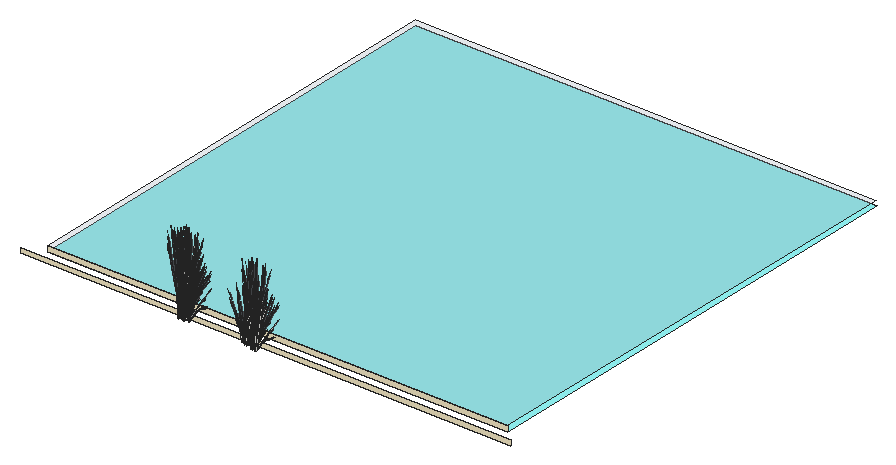
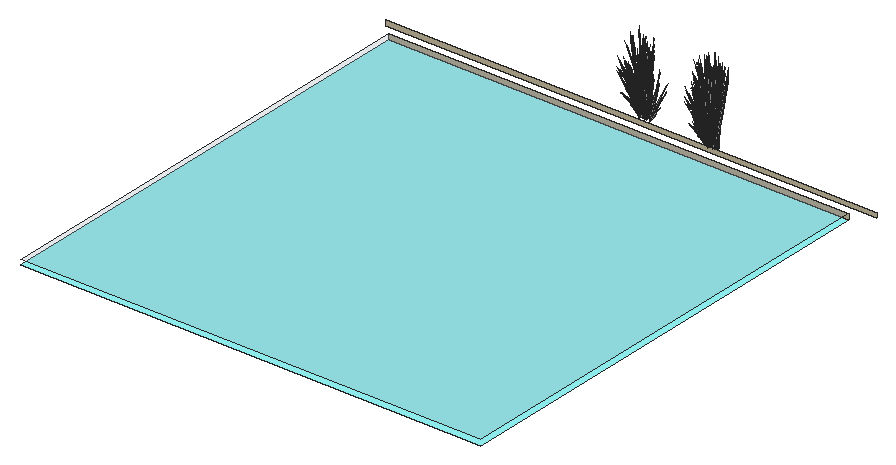
# SketchUp Ruby script. Lengths in inches.
U = 1.inch
M = Sketchup.active_model
def pt(a) = Geom::Point3d.new(a.map { |v| v * U })
def face(e, loops, mat)
  f = e.add_face(loops[0].map { |a| pt(a) })
  loops[1..].each { |l| e.add_face(l.map { |a| pt(a) }).erase! }
  f.material = f.back_material = mat if mat
  f
end
# faces: each face lists its corners as indices into pts; further lists are holes
def faces(e, pts, list, mat = nil) = list.each { |f| face(e, (f[0].is_a?(Array) ? f : [f]).map { |l| l.map { |i| pts[i] } }, mat) }
# xy, xz, yz: faces in a plane at the given z, y or x. An outline is a flat list of corners, or four numbers for a rectangle; further outlines are holes
def ring(l) = l.size == 4 ? [[l[0], l[1]], [l[2], l[1]], [l[2], l[3]], [l[0], l[3]]] : l.each_slice(2).to_a
def flat(e, list, mat, &to3) = list.each { |f| face(e, (f[0].is_a?(Array) ? f : [f]).map { |l| ring(l).map { |u, v| to3.(u, v) } }, mat) }
def xy(e, z, list, mat = nil) = flat(e, list, mat) { |x, y| [x, y, z] }
def xz(e, y, list, mat = nil) = flat(e, list, mat) { |x, z| [x, y, z] }
def yz(e, x, list, mat = nil) = flat(e, list, mat) { |y, z| [x, y, z] }
def lines(e, pts, list) = list.each { |a, b| e.add_line(pt(pts[a]), pt(pts[b])) }
# prism: a flat outline (further loops are holes) pulled along v
def prism(e, loops, v, mat = nil)
  f = face(e, loops, mat); d = Geom::Vector3d.new(v.map { |x| x * U })
  f.pushpull(f.normal.samedirection?(d) ? d.length : -d.length)
end
def box(e, o, s, mat = nil) = prism(e, [[o, [o[0] + s[0], o[1], o[2]], [o[0] + s[0], o[1] + s[1], o[2]], [o[0], o[1] + s[1], o[2]]]], [0, 0, s[2]], mat)
def at(x, y, z, deg = 0) = Geom::Transformation.translation(pt([x, y, z])) * Geom::Transformation.rotation(ORIGIN, Z_AXIS, deg.degrees)
def axes(o, x, y, z) = Geom::Transformation.new([*x, 0, *y, 0, *z, 0, *pt(o).to_a, 1])
def part(name) = M.definitions.add(name)
# library, detail: a bought-in or finely detailed component or shape, given as its bounding box
def library(name, o, s) = part(name).tap { |d| box(d.entities, o, s) }
def detail(e, o, s) = box(e.add_group.entities, o, s)
def put(e, d, t, mat = nil) = e.add_instance(d, t).tap { |i| i.material = mat if mat }
def group(e, t, mat = nil) = e.add_group.tap { |g| g.transformation = t; g.material = mat if mat }.entities
root = M.entities
M.materials.add("D01_Frost_White").color = [255, 242, 206]
M.materials.add("Glass_Basic_01").color = [161, 173, 186]
M.materials["Glass_Basic_01"].alpha = 0.25
M.materials.add("H02_Aqua_Frost").color = [153, 255, 255]
M.materials.add("LightPink_Translucent").color = [144, 107, 117]
M.materials["LightPink_Translucent"].alpha = 0.75
c1 = part("blade")
p = [[2.15,0.21,22],[0,0.17,0],[0.09,0.45,0],[2.18,0.31,22],[2.29,0.31,22],[0.38,0.45,0],
  [2.48,0.24,33],[2.49,0.24,33],[2.48,0.22,33]]
faces(c1.entities,p,[[0,1,2,3],[4,5,2,3],[6,3,4,7],[8,0,3,6]])
c2 = part("seeds")
p = [[0.3,-0.1,1.38],[-0.01,-0.03,1.59],[-0.01,-0.03,0.03],[0.14,-0.07,-0.07],[0.29,-0.03,3],[0.15,0.01,3.11]]
faces(c2.entities,p,[[0,1,2,3],[1,0,4,5]],"LightPink_Translucent")
c3 = part("blade with seeds")
put(c3.entities,c1,at(0,0,0))
put(c3.entities,c2,axes([2.4,0.25,30.99],[1.5799,-0.05474,1.17369],[-0.12525,1.92788,0.29478],[-0.07173,-0.02425,1.56792]))
xy(root,0,[[666.12,288,846,468]],"H02_Aqua_Frost")
xy(root,2,[[666.12,288,846,468]],"Glass_Basic_01")
xz(root,282,[[660.12,0,852,2]],"D01_Frost_White")
xz(root,288,[[666.12,0,846,2]],"D01_Frost_White")
put(root,c3,axes([724.84,280.2,1.22],[0.1218,-0.38743,-0.11714],[0.57753,0.06753,0.25635],[-0.10091,-0.0535,0.7822]))
put(root,c3,axes([753.51,278.125,1.11],[-0.49904,0.02018,-0.2237],[-0.04513,-0.33504,0.10766],[-0.08934,0.03396,0.71822]))
put(root,c3,axes([755.85,278.29,1.3],[-0.11068,-0.08041,0.71501],[0.144,-0.26601,-0.15377],[0.22393,0.03604,0.3057]))
put(root,c3,axes([753.875,278.58,1.1],[0.4633,0.14679,0],[-0.22297,0.30501,0],[0,0,0.87477]))
put(root,c3,axes([724.87,279.54,1.36],[-0.49904,0.02018,0.2237],[-0.04513,-0.33504,-0.10766],[0.08934,-0.03396,0.71822]))
put(root,c3,axes([723.58,279.78,1.24],[0,0.32696,0.24825],[-0.51416,0,0],[0,-0.07447,0.78752]))
put(root,c3,axes([727.21,280.11,2.52],[-0.23123,-0.29606,-0.0608],[0.41039,-0.14549,-0.33747],[0.17294,-0.03906,0.51278]))
put(root,c3,axes([727.19,279.86,2.34],[0.1245,-0.29741,-0.25549],[0.42685,0.10194,-0.1979],[0.17186,-0.02727,0.48886]))
put(root,c3,axes([755.22,278.41,2.36],[0.09858,-0.00553,0.87472],[0.2704,-0.25401,-0.13834],[0.17535,0.03353,0.07015]))
put(root,c3,axes([754.06,278.9,1.1],[-0.28374,-0.32877,-0.02571],[0.4807,-0.18271,0.25804],[-0.11845,0.0313,0.81815]))
put(root,c3,axes([726.52,278.64,1.1875],[0.28732,-0.32763,0],[0.4807,0.18271,-0.25804],[0.10948,0.04161,0.81856]))
put(root,c3,axes([753.96,278.11,1.31],[0.33952,0.19644,0.0724],[-0.2832,0.22163,-0.20674],[-0.07883,0.02996,0.63372]))
put(root,c3,axes([724.8,280.05,1.11],[-0.27607,-0.27443,-0.2237],[0.41817,-0.19325,0.10766],[-0.08934,-0.03396,0.71822]))
put(root,c3,axes([724.85,279.66,1.18],[0.1998,0.3656,0.22877],[-0.5709,0.12713,0.08977],[0.00698,-0.06718,0.79428]))
put(root,c3,axes([751.28,278.16,2.37],[-0.11397,-0.30091,0.24001],[0.44709,-0.05222,0.1979],[-0.13177,0.07077,0.49665]))
put(root,c3,axes([751.1875,278.1,2.37],[-0.31549,-0.13751,0.03215],[0.18368,-0.19581,0.2531],[-0.10115,0.06331,0.38595]))
put(root,c3,axes([751.33,277.74,1.9375],[0.15946,-0.06916,0.85688],[0.13424,0.31957,0.06928],[-0.25033,0.07223,0.36631]))
put(root,c3,axes([727.65,279.9375,0.99],[-0.29599,0.03924,0.70792],[-0.04711,-0.31232,0.04052],[0.20731,-0.04727,0.40283]))
put(root,c3,axes([728.1875,279.66,1.13],[-0.28491,-0.20907,-0.03244],[0.31204,-0.19157,-0.14708],[0.08842,-0.01349,0.48512]))
put(root,c3,axes([724.75,279.95,1.36],[-0.22297,0.29461,0.2237],[-0.4633,-0.14179,-0.10766],[0,-0.06791,0.71822]))
put(root,c3,axes([725.57,279.69,1.1],[0,-0.37831,0],[0.57465,0,0],[0,0,0.89728]))
put(root,c3,axes([754.84,278.45,2.49],[0.45939,0.00787,-0.35523],[-0.03085,0.3315,0.04287],[0.19462,0.03498,0.5025]))
put(root,c3,axes([726.27,278.82,1.24],[-0.4301,-0.16348,0.24825],[0.25708,-0.29314,0],[0.09796,0.03723,0.78752]))
put(root,c3,axes([727.11,279.96,2.49],[0.40382,-0.1444,-0.35523],[0.22505,0.29724,0.04287],[0.19512,-0.03377,0.5025]))
put(root,c3,axes([754.32,278.71,1.24],[0.4301,-0.16348,0.24825],[0.25708,0.29314,0],[-0.09796,0.03723,0.78752]))
put(root,c3,axes([753.71,278.46,1.15],[0.1998,0.37562,-0.03006],[-0.5709,0.13162,0],[0.00698,0.01312,0.86086]))
put(root,c3,axes([753.93,278.86,1.01],[-0.42874,-0.0809,-0.15489],[0.10795,-0.28489,0.15489],[-0.08643,0.03285,0.69487]))
put(root,c3,axes([725.3,279.45,1.18],[-0.38104,0.29672,0.22877],[-0.45269,-0.26192,0.08977],[0.09186,-0.02961,0.79428]))
put(root,c3,axes([750.84,278.28,1.3],[0.15971,0.02684,0.71501],[0.10294,0.27415,-0.15377],[-0.21694,0.05132,0.3057]))
put(root,c3,axes([725.72,279.98,1.15],[-0.42746,-0.28142,-0.03066],[0.42772,-0.28159,0],[-0.01493,-0.00983,0.87786]))
put(root,c3,axes([751.55,278.06,2.53],[0.40003,-0.04673,0.17707],[0.10563,0.26712,-0.2286],[-0.11464,0.07175,0.4374]))
put(root,c3,axes([755.59,277.78,1.1875],[0.57465,0,0],[0,0.36542,-0.25804],[0,0.08323,0.81856]))
put(root,c3,axes([724.64,278.96,1.24],[-0.13276,0.32494,0.08821],[-0.4858,-0.09195,0.17543],[0.08392,-0.00158,0.80203]))
put(root,c3,axes([750.01,277.94,2.35],[0.05865,0.00877,0.88692],[0.18143,0.28888,-0.08381],[-0.12006,0.07582,0.15695]))
put(root,c3,axes([755.36,277.96,1.1],[-0.57436,-0.00261,-0.02488],[0,-0.36542,0.24971],[-0.01805,0.08319,0.79176]))
put(root,c3,axes([727.05,280.02,2.53],[-0.38192,-0.09121,0.17707],[0.11139,-0.2661,-0.2286],[0.15377,-0.0244,0.4374]))
put(root,c3,axes([754.11,277.65,1.33],[0.51755,0.15601,-0.14548],[-0.2492,0.32927,-0.25001],[0.01626,0.08084,0.79854]))
put(root,c3,axes([724.4375,279.23,0.8],[-0.45234,0.1309,0.64464],[-0.14398,-0.37559,0.25048],[0.27777,0.00625,0.73321]))
put(root,c3,axes([750.5,278.86,1.38],[0.19152,-0.14818,0.5743],[0.07557,0.23459,0.42196],[-0.13841,0.042,0.12649]))
put(root,c3,axes([755.11,278.58,2.26],[0.26148,0.20471,-0.17707],[-0.29857,0.19378,0.2286],[0.1517,0.02948,0.4374]))
put(root,c3,axes([725.65,279.32,1.31],[0.08866,-0.29179,0.0724],[0.43315,0.05065,-0.20674],[0.07883,0.02996,0.63372]))
put(root,c3,axes([755.24,278.02,1.01],[-0.32079,0.20399,-0.15489],[-0.32079,-0.20399,0.15489],[0,0.06571,0.69487]))
put(root,c3,axes([753.86,278.04,1.33],[0.05355,0.37308,-0.14548],[-0.55775,0.02256,-0.25001],[-0.09822,0.04969,0.79854]))
put(root,c3,axes([754.98,278.66,2.37],[-0.02314,0.24862,0.03215],[-0.34943,-0.00682,0.2531],[0.13385,0.02602,0.38595]))
put(root,c3,axes([754.06,277.89,1.11],[-0.22297,0.29461,-0.2237],[-0.4633,-0.14179,0.10766],[0,0.06791,0.71822]))
put(root,c3,axes([724.9,280.02,1.18],[0.58084,0.06889,0.22877],[-0.11821,0.38906,0.08977],[-0.08488,-0.03757,0.79428]))
put(root,c3,axes([727.97,279.73,0.75],[-0.02402,-0.04964,0.88171],[0.16658,-0.29036,-0.1347],[0.16804,-0.00418,0.15018]))
put(root,c3,axes([751.23,278.22,2.26],[-0.40003,0.04673,-0.17707],[-0.10563,-0.26712,0.2286],[-0.11464,0.07175,0.4374]))
put(root,c3,axes([755.01,278.58,2.37],[-0.33886,0.21544,0.24001],[-0.29224,-0.22879,0.1979],[0.15898,0.03974,0.49665]))
put(root,c3,axes([725.47,279.4,1.36],[-0.27607,-0.27443,0.2237],[0.41817,-0.19325,-0.10766],[0.08934,0.03396,0.71822]))
put(root,c3,axes([724.04,280.66,1.01],[-0.10795,-0.28489,-0.15489],[0.42874,-0.0809,0.15489],[-0.08643,-0.03285,0.69487]))
put(root,c3,axes([724.59,280.64,1.24],[0.49383,-0.08678,0.08821],[0.12194,0.32295,0.17543],[-0.04404,-0.04705,0.80203]))
put(root,c3,axes([725.61,279.42,1.33],[0.46399,-0.21707,-0.14548],[0.30855,0.30672,-0.25001],[0.11448,0.03115,0.79854]))
put(root,c3,axes([727.45,279.99,2.26],[0.38192,0.09121,-0.17707],[-0.11139,0.2661,0.2286],[0.15377,-0.0244,0.4374]))
put(root,c3,axes([750.64,278.82,2.82],[0.40553,0.08728,-0.03244],[-0.12475,0.26862,-0.14708],[-0.06633,0.04078,0.48512]))
put(root,c3,axes([753.52,278.32,1.03],[-0.30954,0.24575,-0.31177],[-0.38452,-0.22284,-0.08182],[-0.12404,0.0613,0.68817]))
put(root,c3,axes([753.93,278.83,2.53],[-0.07098,-0.26335,0.17707],[0.40574,-0.06954,-0.2286],[0.10898,0.07547,0.4374]))
put(root,c3,axes([726.78,278.84,1.01],[0.4301,0.16348,-0.24825],[-0.25708,0.29314,0],[0.09796,0.03723,0.78752]))
put(root,c3,axes([754.07,278.73,1.17],[0.57533,0.10627,0.15378],[-0.14394,0.37986,-0.18246],[-0.09522,0.04754,0.82443]))
put(root,c3,axes([754.03,278.99,1.01],[-0.4301,0.16348,-0.24825],[-0.25708,-0.29314,0],[-0.09796,0.03723,0.78752]))
put(root,c3,axes([755.46,278.02,1.01],[0,0.32696,-0.24825],[-0.51416,0,0],[0,0.07447,0.78752]))
put(root,c3,axes([725.96,279.77,1.1],[0.51416,0,0],[0,0.33849,0],[0,0,0.89203]))
put(root,c3,axes([754.17,278.06,1.9375],[-0.1707,-0.05633,0.85688],[0.35326,-0.23632,0.06928],[0.22018,0.10661,0.36631]))
put(root,c3,axes([725.09,280.2,1.33],[-0.46399,0.21707,-0.14548],[-0.30855,-0.30672,-0.25001],[-0.11448,-0.03115,0.79854]))
put(root,c3,axes([726.11,278.98,1.24],[-0.49383,0.08678,0.08821],[-0.12194,-0.32295,0.17543],[0.04404,0.04705,0.80203]))
put(root,c3,axes([754.21,277.32,2.24],[-0.39711,-0.16988,0.69141],[0.41931,-0.2645,0.29833],[0.12812,0.1594,0.66832]))
put(root,c3,axes([726.41,279.66,1.9375],[-0.19062,0.00741,0.85688],[0.12645,-0.32094,0.06928],[0.27165,0.01985,0.36631]))
put(root,c3,axes([726.66,278.96,1.01],[0.10795,0.28489,-0.15489],[-0.42874,0.0809,0.15489],[0.08643,0.03285,0.69487]))
put(root,c3,axes([751.34,278.04,2.52],[0.4251,0.18028,-0.0608],[-0.24491,0.26108,-0.33747],[-0.1201,0.09075,0.51278]))
put(root,c3,axes([754.81,278.7,1.38],[-0.25875,-0.09401,0.5743],[0.33411,-0.09552,0.42196],[0.09012,0.08091,0.12649]))
put(root,c3,axes([753.9,278.97,2.52],[0.27385,-0.27986,-0.0608],[0.39658,0.16123,-0.33747],[0.13785,0.07907,0.51278]))
put(root,c3,axes([727.4,280.1,2.37],[0.16879,0.22293,0.03215],[-0.30779,0.10912,0.2531],[0.13568,-0.02153,0.38595]))
put(root,c3,axes([751.92,277.95,1.9375],[0.11478,-0.10046,0.85688],[0.28982,0.27117,0.06928],[-0.19878,0.12349,0.36631]))
put(root,c3,axes([725.8,279.6,1.19],[-0.58084,-0.06889,0.24599],[0.11821,-0.38906,0.09653],[0.08488,0.03757,0.85407]))
put(root,c3,axes([727.36,280.02,2.37],[-0.12984,0.29812,0.24001],[-0.42685,-0.10194,0.1979],[0.16786,-0.01792,0.49665]))
put(root,c3,axes([725.33,280.5625,1.1],[-0.14994,-0.28188,0],[0.42817,-0.09871,0],[0,0,0.77185]))
put(root,c3,axes([751.56,278.25,2.34],[0.11806,0.29854,-0.25549],[-0.44709,0.05222,-0.1979],[-0.12812,0.08019,0.48886]))
put(root,c3,axes([725.05,280.3,1.31],[-0.08866,0.29179,0.0724],[-0.43315,-0.05065,-0.20674],[-0.07883,-0.02996,0.63372]))
put(root,c3,axes([752.09,278.59,2.53],[0.31095,-0.17214,0.17707],[0.29435,0.19656,-0.2286],[-0.04479,0.09987,0.4374]))
put(root,c3,axes([754.42,278.94,1.1875],[0.28732,0.32763,0],[-0.4807,0.18271,-0.25804],[-0.10948,0.04161,0.81856]))
put(root,c3,axes([725.89,280.52,1.09],[0.48247,-0.11094,-0.09599],[0.16954,0.31956,0.00004],[0.05326,-0.01226,0.86949]))
put(root,c3,axes([726.06,280.66,1.24],[0.13276,-0.32494,0.08821],[0.4858,0.09195,0.17543],[-0.08392,0.00158,0.80203]))
put(root,c3,axes([753.54,279.2,2.35],[0.00136,-0.03958,0.88692],[0.39383,-0.17464,-0.08381],[0.1368,0.06234,0.15695]))
put(root,c3,axes([754.88,279.05,0.75],[0.03348,-0.0472,0.88171],[0.42153,-0.13902,-0.1347],[0.12779,0.07195,0.15018]))
put(root,c3,axes([754.18,277.64,1.42],[-0.01255,-0.30784,0.70636],[0.56816,0.0798,0.29908],[-0.13438,0.16845,0.66675]))
put(root,c3,axes([725.95,279.92,1.11],[0.32079,0.21119,0],[-0.32079,0.21119,0],[0,0,0.84633]))
put(root,c3,axes([754.32,277.98,1.05],[0.16851,0.29936,-0.34606],[-0.4854,0.10781,-0.09083],[0.01863,0.10137,0.76386]))
put(root,c3,axes([751.81,278.75,2.37],[-0.37765,-0.01523,0.03215],[0.01035,-0.23004,0.2531],[-0.03952,0.08812,0.38595]))
put(root,c3,axes([751.01,279.01,0.75],[0.06164,0.03267,0.88171],[0.10452,0.30266,-0.1347],[-0.13662,0.06454,0.15018]))
put(root,c3,axes([751.93,278.77,2.37],[-0.32725,-0.22308,0.24001],[0.34753,-0.1924,0.1979],[-0.06036,0.10466,0.49665]))
put(root,c3,axes([754.22,278.83,2.34],[0.45348,-0.07772,-0.25549],[0.07933,0.29434,-0.1979],[0.1218,0.08435,0.48886]))
put(root,c3,axes([726.82,279.83,1.24],[-0.36107,-0.23816,0.08821],[0.36387,-0.231,0.17543],[-0.03988,0.04864,0.80203]))
put(root,c3,axes([726.15,279.47,1.03],[0.47805,0.0536,-0.31177],[-0.10088,0.33065,-0.08182],[0.14266,0.04007,0.68817]))
put(root,c3,axes([728.26,280.05,1.38],[-0.28394,0.05398,0.5743],[0.13365,-0.22308,0.42196],[0.15063,0.01526,0.12649]))
put(root,c3,axes([752.96,278.875,2.53],[0.13855,-0.25143,0.17707],[0.4042,0.07334,-0.2286],[0.03706,0.10123,0.4374]))
put(root,c3,axes([725.23,280.69,1.1],[-0.4633,-0.14679,0],[0.22297,-0.30501,0],[0,0,0.81353]))
put(root,c3,axes([725.61,280.3,1.23],[-0.44875,-0.26316,-0.12596],[0.3776,-0.2955,0.27565],[-0.12084,0.03078,0.84108]))
put(root,c3,axes([724.43,280.8,1.24],[0.4301,0.16348,0.24825],[-0.25708,0.29314,0],[-0.09796,-0.03723,0.78752]))
put(root,c3,axes([754.85,279.13,1.33],[-0.2947,-0.01025,0.5253],[0.19462,-0.21779,0.29003],[0.11642,0.07737,0.41205]))
put(root,c3,axes([725.95,279.67,1.36],[0.22297,-0.29461,0.2237],[0.4633,0.14179,-0.10766],[0,0.06791,0.71822]))
put(root,c3,axes([728.13,280.99,2.35],[-0.04155,-0.02862,0.88692],[0.0909,-0.30682,-0.08381],[0.16368,-0.0196,0.15695]))
put(root,c3,axes([754,279.07,2.37],[-0.20887,0.2077,0.03215],[-0.29744,-0.12092,0.2531],[0.09616,0.06659,0.38595]))
put(root,c3,axes([753.51,279.77,2.82],[0.31757,-0.18757,-0.03244],[0.29098,0.20543,-0.14708],[0.02049,0.05821,0.48512]))
put(root,c3,axes([725.86,279.84,1.15],[0,0.37813,-0.02818],[-0.57465,0,0],[0,0.01188,0.89684]))
put(root,c3,axes([725.9,279.57,1.11],[0.27607,0.27443,-0.2237],[-0.41817,0.19325,0.10766],[0.08934,0.03396,0.71822]))
put(root,c3,axes([754.09,279.01,2.37],[-0.45708,0.07503,0.24001],[-0.07933,-0.29434,0.1979],[0.1075,0.08675,0.49665]))
put(root,c3,axes([727.77,280.73,1.96],[-0.08796,-0.27485,-0.01746],[0.41573,-0.06319,-0.07916],[0.08682,0.01742,0.26109]))
put(root,c3,axes([726.69,280.72,2.52],[0.02461,-0.33251,-0.0608],[0.4659,0.00909,-0.33747],[0.17944,0.0231,0.51278]))
put(root,c3,axes([727.12,279.84,1.24],[0,-0.32696,0.24825],[0.51416,0,0],[0,0.07447,0.78752]))
put(root,c3,axes([751.83,278.2,1.9375],[0.08557,-0.11238,0.85688],[0.35897,0.23257,0.06928],[-0.16194,0.14495,0.36631]))
put(root,c3,axes([725.83,280.08,1.36],[0.49904,-0.02018,0.2237],[0.04513,0.33504,-0.10766],[-0.08934,0.03396,0.71822]))
put(root,c3,axes([726.14,279.74,1.31],[0.42817,-0.09535,0.0724],[0.14994,0.27228,-0.20674],[0,0.05992,0.63372]))
put(root,c3,axes([753.88,278.6,1.3],[0.00811,-0.10838,0.71501],[0.38755,-0.12106,-0.15377],[0.11964,0.12972,0.3057]))
put(root,c3,axes([726.62,280.59,2.53],[-0.26148,-0.20471,0.17707],[0.29857,-0.19378,-0.2286],[0.1517,0.02948,0.4374]))
put(root,c3,axes([725.38,280.24,1.11],[-0.49904,0.02018,-0.2237],[-0.04513,-0.33504,0.10766],[-0.08934,0.03396,0.71822]))
put(root,c3,axes([752.84,279.1,2.37],[-0.33863,0.11112,0.03215],[-0.16575,-0.20263,0.2531],[0.0327,0.08932,0.38595]))
put(root,c3,axes([751.93,278.84,2.26],[-0.31095,0.17214,-0.17707],[-0.29435,-0.19656,0.2286],[-0.04479,0.09987,0.4374]))
put(root,c3,axes([750.86,278.79,2.36],[-0.01142,0.0647,0.87472],[0.32418,0.22509,-0.13834],[-0.08487,0.10644,0.07015]))
put(root,c3,axes([751.89,278.64,2.7],[0.50507,0.0162,-0.06749],[-0.01381,0.30672,-0.3746],[-0.03508,0.11813,0.56919]))
put(root,c3,axes([752.83,278.98,2.52],[0.44971,-0.15222,-0.0608],[0.221,0.27017,-0.33747],[0.05933,0.11385,0.51278]))
put(root,c3,axes([727.73,280.4,1.3],[-0.11068,-0.08041,0.71501],[0.144,-0.26601,-0.15377],[0.22393,0.03604,0.3057]))
put(root,c3,axes([752.96,279.08,2.53],[-0.45283,-0.08548,0.26641],[0.15485,-0.28101,0.21967],[0.02721,0.11051,0.55128]))
put(root,c3,axes([752.13,279.5,1.38],[-0.01189,-0.19441,0.5743],[0.29719,0.13866,0.42196],[-0.05845,0.09266,0.12649]))
put(root,c3,axes([725.75,280.7,1.1],[0.4633,0.14679,0],[-0.22297,0.30501,0],[0,0,0.87477]))
put(root,c3,axes([752.91,279.04,0.75],[0.07437,-0.01779,0.88171],[0.44738,0.09793,-0.1347],[0.01308,0.11037,0.15018]))
put(root,c3,axes([727.1,280.53,2.36],[0.09858,-0.00553,0.87472],[0.2704,-0.25401,-0.13834],[0.17535,0.03353,0.07015]))
put(root,c3,axes([725.9375,281.02,1.1],[-0.28374,-0.32877,-0.02571],[0.4807,-0.18271,0.25804],[-0.11845,0.0313,0.81815]))
put(root,c3,axes([725.84,280.23,1.31],[0.33952,0.19644,0.0724],[-0.2832,0.22163,-0.20674],[-0.07883,0.02996,0.63372]))
put(root,c3,axes([752.24,278.75,2.5],[0.32898,0.21969,-0.2836],[-0.34753,0.1924,-0.21967],[-0.05006,0.11162,0.54264]))
put(root,c3,axes([751.88,279.08,1.41],[0.41748,-0.0579,0.03254],[0.09598,0.23326,-0.43152],[-0.02647,0.11808,0.3868]))
put(root,c3,axes([753.21,278.97,2.34],[0.45175,0.08196,-0.25549],[-0.15485,0.28101,-0.1979],[0.04142,0.11314,0.48886]))
put(root,c3,axes([753.47,278.39,1.9375],[-0.10505,-0.10498,0.85688],[0.48542,-0.08838,0.06928],[0.10971,0.1648,0.36631]))
put(root,c3,axes([726.71,280.56,2.49],[0.45939,0.00787,-0.35523],[-0.03085,0.3315,0.04287],[0.19462,0.03498,0.5025]))
put(root,c3,axes([753.01,279.14,2.26],[-0.13855,0.25143,-0.17707],[-0.4042,-0.07334,0.2286],[0.03706,0.10123,0.4374]))
put(root,c3,axes([726.2,280.83,1.24],[0.4301,-0.16348,0.24825],[0.25708,0.29314,0],[-0.09796,0.03723,0.78752]))
put(root,c3,axes([725.59,280.57,1.15],[0.1998,0.37562,-0.03006],[-0.5709,0.13162,0],[0.00698,0.01312,0.86086]))
put(root,c3,axes([725.81,280.98,1.01],[-0.42874,-0.0809,-0.15489],[0.10795,-0.28489,0.15489],[-0.08643,0.03285,0.69487]))
put(root,c3,axes([752.14,278.65,2.67],[-0.01196,0.30243,-0.3943],[-0.50354,-0.02031,0.04758],[-0.05314,0.12813,0.55778]))
put(root,c3,axes([750.82,279.45,2.35],[0.05214,-0.01974,0.88692],[0.43092,0.1313,-0.08381],[-0.01013,0.10932,0.15695]))
put(root,c3,axes([727.46,279.89,1.1875],[0.57465,0,0],[0,0.36542,-0.25804],[0,0.08323,0.81856]))
put(root,c3,axes([727.24,280.08,1.1],[-0.57436,-0.00261,-0.02488],[0,-0.36542,0.24971],[-0.01805,0.08319,0.79176]))
put(root,c3,axes([752.61,278.44,1.9375],[-0.01125,-0.12549,0.85688],[0.48751,0.08325,0.06928],[-0.03015,0.17883,0.36631]))
put(root,c3,axes([725.99,279.76,1.33],[0.51755,0.15601,-0.14548],[-0.2492,0.32927,-0.25001],[0.01626,0.08084,0.79854]))
put(root,c3,axes([726.99,280.7,2.26],[0.26148,0.20471,-0.17707],[-0.29857,0.19378,0.2286],[0.1517,0.02948,0.4374]))
put(root,c3,axes([727.12,280.13,1.01],[-0.32079,0.20399,-0.15489],[-0.32079,-0.20399,0.15489],[0,0.06571,0.69487]))
put(root,c3,axes([725.73,280.15,1.33],[0.05355,0.37308,-0.14548],[-0.55775,0.02256,-0.25001],[-0.09822,0.04969,0.79854]))
put(root,c3,axes([726.86,280.78,2.37],[-0.02314,0.24862,0.03215],[-0.34943,-0.00682,0.2531],[0.13385,0.02602,0.38595]))
put(root,c3,axes([725.9375,280.01,1.11],[-0.22297,0.29461,-0.2237],[-0.4633,-0.14179,0.10766],[0,0.06791,0.71822]))
put(root,c3,axes([753.05,278.91,2.49],[0.21934,0.26585,-0.35523],[-0.45151,0.14816,0.04287],[0.05129,0.12845,0.5025]))
put(root,c3,axes([726.89,280.7,2.37],[-0.33886,0.21544,0.24001],[-0.29224,-0.22879,0.1979],[0.15898,0.03974,0.49665]))
put(root,c3,axes([751.78,279.33,1.3],[0.14502,-0.05158,0.71501],[0.35805,0.15552,-0.15377],[-0.10657,0.13457,0.3057]))
put(root,c3,axes([752.72,279.59,2.36],[0.05825,0.05265,0.87472],[0.47011,0.02068,-0.13834],[0.04727,0.11612,0.07015]))
put(root,c3,axes([725.4,280.4375,1.03],[-0.30954,0.24575,-0.31177],[-0.38452,-0.22284,-0.08182],[-0.12404,0.0613,0.68817]))
put(root,c3,axes([725.8125,280.95,2.53],[-0.07098,-0.26335,0.17707],[0.40574,-0.06954,-0.2286],[0.10898,0.07547,0.4374]))
put(root,c3,axes([725.95,280.85,1.17],[0.57533,0.10627,0.15378],[-0.14394,0.37986,-0.18246],[-0.09522,0.04754,0.82443]))
put(root,c3,axes([725.91,281.11,1.01],[-0.4301,0.16348,-0.24825],[-0.25708,-0.29314,0],[-0.09796,0.03723,0.78752]))
put(root,c3,axes([727.34,280.14,1.01],[0,0.32696,-0.24825],[-0.51416,0,0],[0,0.07447,0.78752]))
put(root,c3,axes([726.05,280.18,1.9375],[-0.1707,-0.05633,0.85688],[0.35326,-0.23632,0.06928],[0.22018,0.10661,0.36631]))
put(root,c3,axes([726.08,279.44,2.24],[-0.39711,-0.16988,0.69141],[0.41931,-0.2645,0.29833],[0.12812,0.1594,0.66832]))
put(root,c3,axes([751.97,279.08,1.68],[0.0101,-0.16879,0.77173],[0.45413,0.08915,0.10664],[-0.03935,0.17989,0.36441]))
put(root,c3,axes([726.68,280.82,1.38],[-0.25875,-0.09401,0.5743],[0.33411,-0.09552,0.42196],[0.09012,0.08091,0.12649]))
put(root,c3,axes([725.77,281.09,2.52],[0.27385,-0.27986,-0.0608],[0.39658,0.16123,-0.33747],[0.13785,0.07907,0.51278]))
put(root,c3,axes([723.97,280.71,2.53],[0.31095,-0.17214,0.17707],[0.29435,0.19656,-0.2286],[-0.04479,0.09987,0.4374]))
put(root,c3,axes([726.3,281.06,1.1875],[0.28732,0.32763,0],[-0.4807,0.18271,-0.25804],[-0.10948,0.04161,0.81856]))
put(root,c3,axes([725.42,281.32,2.35],[0.00136,-0.03958,0.88692],[0.39383,-0.17464,-0.08381],[0.1368,0.06234,0.15695]))
put(root,c3,axes([726.76,281.17,0.75],[0.03348,-0.0472,0.88171],[0.42153,-0.13902,-0.1347],[0.12779,0.07195,0.15018]))
put(root,c3,axes([726.05,279.76,1.42],[-0.01255,-0.30784,0.70636],[0.56816,0.0798,0.29908],[-0.13438,0.16845,0.66675]))
put(root,c3,axes([726.2,280.1,1.05],[0.16851,0.29936,-0.34606],[-0.4854,0.10781,-0.09083],[0.01863,0.10137,0.76386]))
put(root,c3,axes([723.6875,280.86,2.37],[-0.37765,-0.01523,0.03215],[0.01035,-0.23004,0.2531],[-0.03952,0.08812,0.38595]))
put(root,c3,axes([723.81,280.89,2.37],[-0.32725,-0.22308,0.24001],[0.34753,-0.1924,0.1979],[-0.06036,0.10466,0.49665]))
put(root,c3,axes([726.1,280.95,2.34],[0.45348,-0.07772,-0.25549],[0.07933,0.29434,-0.1979],[0.1218,0.08435,0.48886]))
put(root,c3,axes([724.84,280.99,2.53],[0.13855,-0.25143,0.17707],[0.4042,0.07334,-0.2286],[0.03706,0.10123,0.4374]))
put(root,c3,axes([726.72,281.25,1.33],[-0.2947,-0.01025,0.5253],[0.19462,-0.21779,0.29003],[0.11642,0.07737,0.41205]))
put(root,c3,axes([725.875,281.1875,2.37],[-0.20887,0.2077,0.03215],[-0.29744,-0.12092,0.2531],[0.09616,0.06659,0.38595]))
put(root,c3,axes([725.39,281.89,2.82],[0.31757,-0.18757,-0.03244],[0.29098,0.20543,-0.14708],[0.02049,0.05821,0.48512]))
put(root,c3,axes([725.96,281.13,2.37],[-0.45708,0.07503,0.24001],[-0.07933,-0.29434,0.1979],[0.1075,0.08675,0.49665]))
put(root,c3,axes([725.76,280.72,1.3],[0.00811,-0.10838,0.71501],[0.38755,-0.12106,-0.15377],[0.11964,0.12972,0.3057]))
put(root,c3,axes([724.72,281.22,2.37],[-0.33863,0.11112,0.03215],[-0.16575,-0.20263,0.2531],[0.0327,0.08932,0.38595]))
put(root,c3,axes([723.81,280.95,2.26],[-0.31095,0.17214,-0.17707],[-0.29435,-0.19656,0.2286],[-0.04479,0.09987,0.4374]))
put(root,c3,axes([723.77,280.76,2.7],[0.50507,0.0162,-0.06749],[-0.01381,0.30672,-0.3746],[-0.03508,0.11813,0.56919]))
put(root,c3,axes([724.71,281.1,2.52],[0.44971,-0.15222,-0.0608],[0.221,0.27017,-0.33747],[0.05933,0.11385,0.51278]))
put(root,c3,axes([724.84,281.2,2.53],[-0.45283,-0.08548,0.26641],[0.15485,-0.28101,0.21967],[0.02721,0.11051,0.55128]))
put(root,c3,axes([724,281.62,1.38],[-0.01189,-0.19441,0.5743],[0.29719,0.13866,0.42196],[-0.05845,0.09266,0.12649]))
put(root,c3,axes([724.79,281.16,0.75],[0.07437,-0.01779,0.88171],[0.44738,0.09793,-0.1347],[0.01308,0.11037,0.15018]))
put(root,c3,axes([724.12,280.87,2.5],[0.32898,0.21969,-0.2836],[-0.34753,0.1924,-0.21967],[-0.05006,0.11162,0.54264]))
put(root,c3,axes([723.76,281.2,1.41],[0.41748,-0.0579,0.03254],[0.09598,0.23326,-0.43152],[-0.02647,0.11808,0.3868]))
put(root,c3,axes([725.09,281.08,2.34],[0.45175,0.08196,-0.25549],[-0.15485,0.28101,-0.1979],[0.04142,0.11314,0.48886]))
put(root,c3,axes([725.35,280.5,1.9375],[-0.10505,-0.10498,0.85688],[0.48542,-0.08838,0.06928],[0.10971,0.1648,0.36631]))
put(root,c3,axes([724.89,281.26,2.26],[-0.13855,0.25143,-0.17707],[-0.4042,-0.07334,0.2286],[0.03706,0.10123,0.4374]))
put(root,c3,axes([724.01,280.77,2.67],[-0.01196,0.30243,-0.3943],[-0.50354,-0.02031,0.04758],[-0.05314,0.12813,0.55778]))
put(root,c3,axes([722.7,281.57,2.35],[0.05214,-0.01974,0.88692],[0.43092,0.1313,-0.08381],[-0.01013,0.10932,0.15695]))
put(root,c3,axes([724.49,280.56,1.9375],[-0.01125,-0.12549,0.85688],[0.48751,0.08325,0.06928],[-0.03015,0.17883,0.36631]))
put(root,c3,axes([724.93,281.03,2.49],[0.21934,0.26585,-0.35523],[-0.45151,0.14816,0.04287],[0.05129,0.12845,0.5025]))
put(root,c3,axes([724.6,281.7,2.36],[0.05825,0.05265,0.87472],[0.47011,0.02068,-0.13834],[0.04727,0.11612,0.07015]))
put(root,c3,axes([723.85,281.2,1.68],[0.0101,-0.16879,0.77173],[0.45413,0.08915,0.10664],[-0.03935,0.17989,0.36441]))
